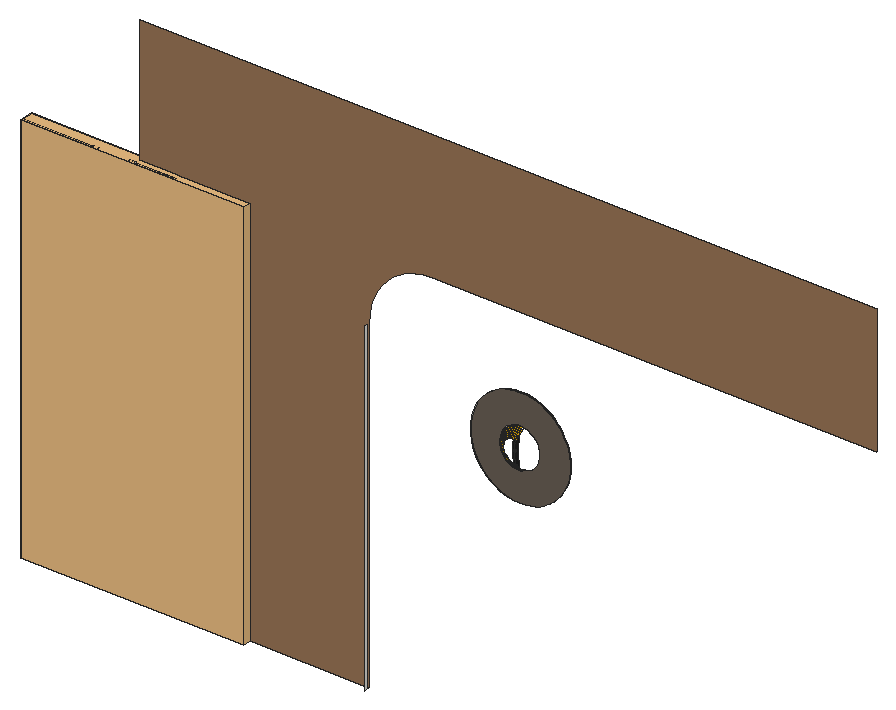
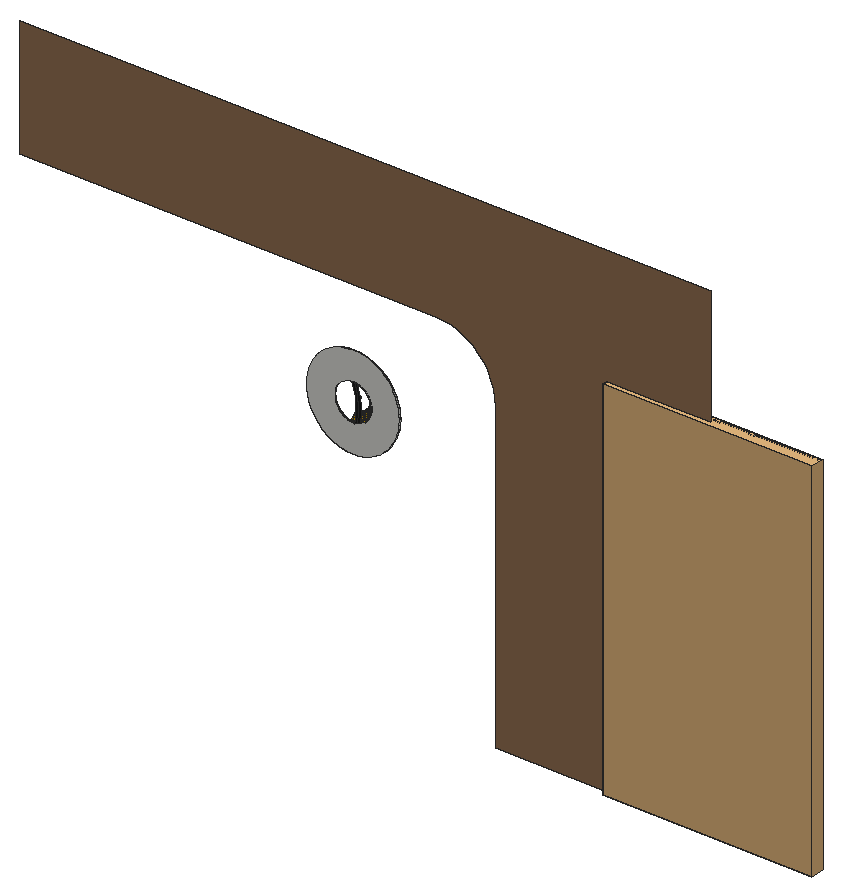
# SketchUp Ruby script. Lengths in inches.
U = 1.inch
M = Sketchup.active_model
def pt(a) = Geom::Point3d.new(a.map { |v| v * U })
def face(e, loops, mat)
  f = e.add_face(loops[0].map { |a| pt(a) })
  loops[1..].each { |l| e.add_face(l.map { |a| pt(a) }).erase! }
  f.material = f.back_material = mat if mat
  f
end
# faces: each face lists its corners as indices into pts; further lists are holes
def faces(e, pts, list, mat = nil) = list.each { |f| face(e, (f[0].is_a?(Array) ? f : [f]).map { |l| l.map { |i| pts[i] } }, mat) }
# xy, xz, yz: faces in a plane at the given z, y or x. An outline is a flat list of corners, or four numbers for a rectangle; further outlines are holes
def ring(l) = l.size == 4 ? [[l[0], l[1]], [l[2], l[1]], [l[2], l[3]], [l[0], l[3]]] : l.each_slice(2).to_a
def flat(e, list, mat, &to3) = list.each { |f| face(e, (f[0].is_a?(Array) ? f : [f]).map { |l| ring(l).map { |u, v| to3.(u, v) } }, mat) }
def xy(e, z, list, mat = nil) = flat(e, list, mat) { |x, y| [x, y, z] }
def xz(e, y, list, mat = nil) = flat(e, list, mat) { |x, z| [x, y, z] }
def yz(e, x, list, mat = nil) = flat(e, list, mat) { |y, z| [x, y, z] }
def lines(e, pts, list) = list.each { |a, b| e.add_line(pt(pts[a]), pt(pts[b])) }
# prism: a flat outline (further loops are holes) pulled along v
def prism(e, loops, v, mat = nil)
  f = face(e, loops, mat); d = Geom::Vector3d.new(v.map { |x| x * U })
  f.pushpull(f.normal.samedirection?(d) ? d.length : -d.length)
end
def box(e, o, s, mat = nil) = prism(e, [[o, [o[0] + s[0], o[1], o[2]], [o[0] + s[0], o[1] + s[1], o[2]], [o[0], o[1] + s[1], o[2]]]], [0, 0, s[2]], mat)
def at(x, y, z, deg = 0) = Geom::Transformation.translation(pt([x, y, z])) * Geom::Transformation.rotation(ORIGIN, Z_AXIS, deg.degrees)
def axes(o, x, y, z) = Geom::Transformation.new([*x, 0, *y, 0, *z, 0, *pt(o).to_a, 1])
def part(name) = M.definitions.add(name)
# library, detail: a bought-in or finely detailed component or shape, given as its bounding box
def library(name, o, s) = part(name).tap { |d| box(d.entities, o, s) }
def detail(e, o, s) = box(e.add_group.entities, o, s)
def put(e, d, t, mat = nil) = e.add_instance(d, t).tap { |i| i.material = mat if mat }
def group(e, t, mat = nil) = e.add_group.tap { |g| g.transformation = t; g.material = mat if mat }.entities
root = M.entities
M.materials.add("Screen Shot 2016-03-02 at 11.42.45 AM").color = [104, 95, 84]
M.materials.add("[0129_WhiteSmoke]").color = [245, 245, 245]
M.materials.add("[0130_Gainsboro]").color = [220, 220, 220]
M.materials.add("[Color D06]").color = [204, 153, 0]
M.materials.add("[Color M08]").color = [30, 30, 30]
M.materials.add("[Wood Floor]").color = [153, 117, 86]
c1 = library("Group\#223",[-0.5,-0.5,0],[45.61,2.875,80.22])
xz(root,755.25,[[[107.55,91.99,108.61,92.04,109.66,92.21,110.6875,92.48,111.68,92.86,112.63,93.35,113.52,93.92,114.34,94.59,115.1,95.34,115.76,96.17,116.34,97.0625,116.83,98.01,117.21,99,117.48,100.03,117.65,101.08,117.7,102.14,117.65,103.2,117.48,104.25,117.21,105.28,116.83,106.27,116.34,107.21,115.76,108.11,115.1,108.93,114.34,109.68,113.52,110.35,112.63,110.93,111.68,111.41,110.6875,111.79,109.66,112.07,108.61,112.24,107.55,112.29,106.49,112.24,105.44,112.07,104.41,111.79,103.42,111.41,102.47,110.93,101.58,110.35,100.76,109.68,100.01,108.93,99.34,108.11,98.76,107.21,98.28,106.27,97.89,105.28,97.62,104.25,97.45,103.2,97.4,102.14,97.45,101.08,97.62,100.03,97.89,99,98.28,98.01,98.76,97.0625,99.34,96.17,100.01,95.34,100.76,94.59,101.58,93.92,102.47,93.35,103.42,92.86,104.41,92.48,105.44,92.21,106.49,92.04],[107.55,98.08,107.125,98.1,106.71,98.17,106.3,98.28,105.9,98.43,105.52,98.62,105.16,98.85,104.83,99.12,104.53,99.42,104.26,99.75,104.03,100.11,103.84,100.49,103.6875,100.88,103.58,101.29,103.51,101.71,103.49,102.14,103.51,102.5625,103.58,102.98,103.6875,103.39,103.84,103.79,104.03,104.17,104.26,104.53,104.53,104.86,104.83,105.16,105.16,105.42,105.52,105.66,105.9,105.85,106.3,106,106.71,106.11,107.125,106.18,107.55,106.2,107.98,106.18,108.39,106.11,108.81,106,109.2,105.85,109.58,105.66,109.9375,105.42,110.27,105.16,110.57,104.86,110.84,104.53,111.07,104.17,111.26,103.79,111.41,103.39,111.52,102.98,111.59,102.5625,111.61,102.14,111.59,101.71,111.52,101.29,111.41,100.88,111.26,100.49,111.07,100.11,110.84,99.75,110.57,99.42,110.27,99.12,109.9375,98.85,109.58,98.62,109.2,98.43,108.81,98.28,108.39,98.17,107.98,98.1]]],"Screen Shot 2016-03-02 at 11.42.45 AM")
xz(root,755.5,[[[107.55,91.99,108.61,92.04,108.73,92.06,109.14,92.125,109.66,92.21,109.77,92.24,110.6875,92.48,111.68,92.86,112.63,93.35,113.4,93.85,113.52,93.92,114.05,94.36,114.34,94.59,115.1,95.34,115.76,96.17,116.34,97.0625,116.83,98.01,117.21,99,117.48,100.03,117.65,101.08,117.7,102.14,117.65,103.2,117.48,104.25,117.21,105.28,116.83,106.27,116.34,107.21,115.76,108.11,115.19,108.8125,115.1,108.93,114.62,109.41,114.34,109.68,113.52,110.35,112.63,110.93,111.68,111.41,111.28,111.57,110.69,111.79,110.6875,111.79,110.29,111.9,109.66,112.07,108.61,112.24,107.55,112.29,106.49,112.24,105.44,112.07,104.41,111.79,103.42,111.41,102.47,110.93,101.58,110.35,100.76,109.68,100.01,108.93,99.34,108.11,98.76,107.21,98.28,106.27,97.89,105.28,97.62,104.25,97.45,103.2,97.4,102.14,97.45,101.08,97.62,100.03,97.89,99,98.28,98.01,98.76,97.0625,99.34,96.17,100.01,95.34,100.76,94.59,101.58,93.92,102.47,93.35,103.42,92.86,104.41,92.48,105.44,92.21,106.49,92.04],[107.55,98.08,107.14,98.1,107.125,98.1,106.71,98.17,106.53,98.21,106.3,98.28,106.125,98.34,105.9,98.43,105.52,98.62,105.16,98.85,104.83,99.12,104.53,99.42,104.26,99.75,104.03,100.11,103.84,100.49,103.6875,100.88,103.58,101.29,103.51,101.71,103.49,102.14,103.51,102.5625,103.58,102.98,103.6875,103.39,103.84,103.79,104.03,104.17,104.26,104.53,104.53,104.86,104.83,105.16,105.16,105.42,105.52,105.66,105.9,105.85,106.3,106,106.71,106.11,106.75,106.12,107.125,106.18,107.16,106.18,107.55,106.2,107.76,106.1875,107.98,106.18,108.39,106.11,108.81,106,109.2,105.85,109.58,105.66,109.9375,105.42,110.27,105.16,110.57,104.86,110.84,104.53,111.07,104.17,111.26,103.79,111.41,103.39,111.52,102.98,111.57,102.66,111.62,102.65,111.59,102.46,111.61,102.14,111.59,101.71,111.52,101.29,111.5,101.21,111.41,100.88,111.26,100.49,111.07,100.11,110.84,99.75,110.76,99.65,110.57,99.42,110.27,99.12,109.9375,98.85,109.58,98.62,109.2,98.43,108.81,98.28,108.39,98.17,107.98,98.1]]])
xz(root,755.5,[[6,46.28,19.81,126.5],[20.99,46.28,27.26,126.5]],"[0129_WhiteSmoke]")
xz(root,755.5,[[28.49,46.28,50.61,46.28,50.61,111.88,50.49,113.79,50.11,115.67,49.5,117.48,48.65,119.19,47.59,120.78,46.33,122.22,44.89,123.48,43.3,124.54,41.59,125.39,39.77,126.01,37.9,126.38,35.99,126.5,28.49,126.5]],"[0130_Gainsboro]")
xz(root,755.5,[[108.73,92.06,109.14,92.125,108.67,92.78,107.875,94.17,107.23,95.63,106.75,97.15,106.53,98.21,106.3,98.28,106.125,98.34,106.39,97.06,106.89,95.5,107.55,94,108.36,92.58],[109.14,92.125,109.66,92.21,109.77,92.24,109.15,93.09,108.39,94.43,107.77,95.84,107.3,97.3,107.14,98.1,107.125,98.1,106.71,98.17,106.53,98.21,106.75,97.15,107.23,95.63,107.875,94.17,108.67,92.78],[107.125,98.1,107.14,98.1,106.99,98.81,106.84,100.34,106.84,101.87,107.01,103.4,107.34,104.9,107.76,106.1875,107.55,106.2,107.16,106.18,106.78,105.05,106.44,103.49,106.27,101.91,106.26,100.31,106.42,98.72,106.53,98.21,106.71,98.17],[106.53,98.21,106.42,98.72,106.26,100.31,106.27,101.91,106.44,103.49,106.78,105.05,107.16,106.18,107.125,106.18,106.75,106.12,106.43,105.15,106.08,103.55,105.9,101.93,105.89,100.29,106.06,98.66,106.125,98.34,106.3,98.28]],"[Color M08]")
xz(root,755.8125,[[19.81,46.28,20.99,126.5],[27.26,46.28,28.49,126.5]],"[Color D06]")
xz(root,756.6875,[[50.61,46.28,75.46,46.28,75.46,113.03,75.57,114.73,75.9,116.39,76.45,118,77.2,119.53,78.14,120.94,79.26,122.22,80.54,123.34,81.96,124.29,83.48,125.04,85.09,125.59,86.76,125.92,88.46,126.03,179.22,126.03,179.22,152.12,28.49,152.12,28.49,126.5,35.99,126.5,37.9,126.38,39.77,126.01,41.59,125.39,43.3,124.54,44.89,123.48,46.33,122.22,47.59,120.78,48.65,119.19,49.5,117.48,50.11,115.67,50.49,113.79,50.61,111.88]],"[Wood Floor]")
yz(root,19.81,[[755.5,46.28,755.8125,126.5]])
yz(root,20.99,[[755.5,46.28,755.8125,126.5]])
yz(root,27.26,[[755.5,46.28,755.8125,126.5]])
yz(root,28.49,[[755.5,46.28,755.8125,126.5]])
yz(root,75.46,[[755.5,46.28,756.09,113.03]])
p = [[105.44,755.5,92.21],[106.49,755.5,92.04],[106.49,755.25,92.04],[105.44,755.25,92.21],[107.55,755.5,91.99],[107.55,755.25,91.99],
  [108.61,755.5,92.04],[108.61,755.25,92.04],[104.41,755.5,92.48],[104.41,755.25,92.48],[103.42,755.5,92.86],[103.42,755.25,92.86],
  [102.47,755.5,93.35],[102.47,755.25,93.35],[101.58,755.5,93.92],[101.58,755.25,93.92],[100.76,755.5,94.59],[100.76,755.25,94.59],
  [100.01,755.5,95.34],[100.01,755.25,95.34],[99.34,755.5,96.17],[99.34,755.25,96.17],[98.76,755.5,97.0625],[98.76,755.25,97.0625],
  [98.28,755.5,98.01],[98.28,755.25,98.01],[97.89,755.5,99],[97.89,755.25,99],[107.125,755.25,98.1],[107.15,754.91,98.3],
  [106.75,754.91,98.37],[106.71,755.25,98.17],[107.55,755.25,98.08],[107.55,754.91,98.28],[107.98,755.25,98.1],[107.95,754.91,98.3],
  [107.125,755.5,98.1],[106.71,755.5,98.17],[107.55,755.5,98.08],[107.14,755.5,98.1],[107.98,755.5,98.1],[106.36,754.91,98.47],
  [106.3,755.25,98.28],[106.53,755.5,98.21],[106.3,755.5,98.28],[107.17,754.6,98.55],[106.8,754.6,98.61],[107.55,754.6,98.53],
  [107.93,754.6,98.55],[108.35,754.91,98.37],[108.3,754.6,98.61],[105.98,754.91,98.62],[105.9,755.25,98.43],[106.125,755.5,98.34],
  [105.9,755.5,98.43],[106.44,754.6,98.71],[105.62,754.91,98.8],[105.52,755.25,98.62],[105.52,755.5,98.62],[107.2,754.33,98.83],
  [106.86,754.33,98.88],[107.55,754.33,98.8125],[107.9,754.33,98.83],[108.24,754.33,98.88],[106.08,754.6,98.84],[106.52,754.33,98.97],
  [105.75,754.6,99.01],[105.28,754.91,99.02],[105.16,755.25,98.85],[105.16,755.5,98.85],[106.2,754.33,99.1],[107.24,754.09,99.14],
  [106.92,754.09,99.19],[107.55,754.09,99.125],[107.87,754.09,99.14],[108.18,754.09,99.19],[105.89,754.33,99.26],[105.43,754.6,99.22],
  [106.62,754.09,99.27],[104.97,754.91,99.27],[104.83,755.25,99.12],[104.83,755.5,99.12],[106.33,754.09,99.39],[105.6,754.33,99.45],
  [105.14,754.6,99.46],[97.62,755.5,100.03],[97.62,755.25,100.03],[107.27,753.9,99.48],[107,753.9,99.53],[107.55,753.9,99.47],
  [107.83,753.9,99.48],[108.11,753.9,99.53],[106.04,754.09,99.53],[104.69,754.91,99.56],[104.53,755.25,99.42],[104.53,755.5,99.42],
  [106.73,753.9,99.6],[105.32,754.33,99.67],[106.46,753.9,99.7],[105.78,754.09,99.7],[104.87,754.6,99.72],[106.22,753.9,99.83],
  [105.54,754.09,99.9],[104.43,754.91,99.87],[104.26,755.25,99.75],[104.26,755.5,99.75],[107.07,753.75,99.88],[106.84,753.75,99.94],
  [107.31,753.75,99.84],[107.55,753.75,99.83],[107.79,753.75,99.84],[108.03,753.75,99.88],[105.98,753.9,99.98],[105.08,754.33,99.91],
  [106.61,753.75,100.03],[104.63,754.6,100.02],[106.4,753.75,100.14],[105.76,753.9,100.15],[105.3125,754.09,100.12],[104.86,754.33,100.18],
  [106.19,753.75,100.27],[104.21,754.91,100.21],[104.03,755.25,100.11],[104.03,755.5,100.11],[105.57,753.9,100.35],[105.11,754.09,100.37],
  [104.42,754.6,100.33],[106.01,753.75,100.42],[104.67,754.33,100.47],[97.45,755.5,101.08],[97.45,755.25,101.08],[105.39,753.9,100.57],
  [104.03,754.91,100.57],[103.84,755.25,100.49],[103.84,755.5,100.49],[105.84,753.75,100.59],[104.94,754.09,100.63],[104.25,754.6,100.67],
  [104.51,754.33,100.78],[105.68,753.75,100.78],[105.24,753.9,100.8],[104.8,754.09,100.91],[103.88,754.91,100.95],[103.6875,755.25,100.88],
  [103.6875,755.5,100.88],[105.55,753.75,100.98],[105.11,753.9,101.05],[104.12,754.6,101.02],[104.39,754.33,101.11],[105.44,753.75,101.2],
  [104.6875,754.09,101.21],[105.01,753.9,101.3125],[104.02,754.6,101.39],[103.78,754.91,101.34],[103.58,755.25,101.29],[103.58,755.5,101.29],
  [104.3,754.33,101.45],[105.36,753.75,101.43],[104.6,754.09,101.51],[97.4,755.5,102.14],[97.4,755.25,102.14],[104.9375,753.9,101.58],
  [105.29,753.75,101.66],[103.96,754.6,101.76],[103.72,754.91,101.74],[103.51,755.25,101.71],[103.51,755.5,101.71],[104.55,754.09,101.82],
  [104.24,754.33,101.79],[104.89,753.9,101.86],[105.26,753.75,101.9],[103.94,754.6,102.14],[103.69,754.91,102.14],[103.49,755.25,102.14],
  [103.49,755.5,102.14],[104.88,753.9,102.14],[104.54,754.09,102.14],[104.22,754.33,102.14],[105.24,753.75,102.14],[105.26,753.75,102.38],
  [104.89,753.9,102.42],[107.18,753.71,102.14],[107.55,753.85,102.14],[107.18,753.71,102.18],[107.19,753.71,102.21],[107.2,753.71,102.25],
  [107.21,753.71,102.29],[107.23,753.71,102.32],[107.25,753.71,102.35],[107.28,753.71,102.38],[107.3,753.71,102.41],[107.33,753.71,102.4375],
  [107.37,753.71,102.46],[107.4,753.71,102.47],[107.4375,753.71,102.49],[107.47,753.71,102.5],[107.51,753.71,102.5],[107.55,753.71,102.51],
  [107.73,753.71,102.46],[107.77,753.71,102.4375],[107.8,753.71,102.41],[107.82,753.71,102.38],[107.85,753.71,102.35],[107.87,753.71,102.32],
  [107.89,753.71,102.29],[107.9,753.71,102.25],[107.91,753.71,102.21],[107.92,753.71,102.18],[107.92,753.71,102.14],[104.55,754.09,102.45],
  [104.24,754.33,102.49],[103.96,754.6,102.52],[103.72,754.91,102.54],[103.51,755.25,102.5625],[97.45,755.5,103.2],[97.45,755.25,103.2],
  [103.51,755.5,102.5625],[105.29,753.75,102.62],[104.9375,753.9,102.69],[104.6,754.09,102.76],[104.3,754.33,102.83],[104.02,754.6,102.89],
  [103.78,754.91,102.94],[103.58,755.25,102.98],[105.36,753.75,102.85],[105.01,753.9,102.96],[103.58,755.5,102.98],[104.6875,754.09,103.07],
  [104.39,754.33,103.17],[104.12,754.6,103.25],[105.44,753.75,103.08],[105.11,753.9,103.22],[103.88,754.91,103.33],[103.6875,755.25,103.39],
  [104.8,754.09,103.36],[103.6875,755.5,103.39],[105.55,753.75,103.29],[105.24,753.9,103.47],[104.51,754.33,103.49],[104.94,754.09,103.64],
  [104.25,754.6,103.61],[97.62,755.5,104.25],[97.62,755.25,104.25],[105.68,753.75,103.49],[105.39,753.9,103.71],[104.03,754.91,103.71],
  [103.84,755.25,103.79],[104.67,754.33,103.8],[103.84,755.5,103.79],[105.84,753.75,103.68],[105.57,753.9,103.92],[105.11,754.09,103.91],
  [104.42,754.6,103.94],[104.86,754.33,104.09],[104.21,754.91,104.07],[106.01,753.75,103.85],[105.76,753.9,104.12],[105.3125,754.09,104.15],
  [104.03,755.25,104.17],[104.63,754.6,104.26],[104.03,755.5,104.17],[106.19,753.75,104],[105.98,753.9,104.3],[105.54,754.09,104.375],
  [105.08,754.33,104.36],[104.43,754.91,104.4],[106.4,753.75,104.14],[106.22,753.9,104.45],[106.61,753.75,104.25],[106.46,753.9,104.58],
  [105.78,754.09,104.57],[104.87,754.6,104.55],[104.26,755.25,104.53],[106.84,753.75,104.33],[106.73,753.9,104.68],[105.32,754.33,104.61],
  [97.89,755.5,105.28],[97.89,755.25,105.28],[104.26,755.5,104.53],[107.07,753.75,104.39],[107,753.9,104.75],[106.04,754.09,104.75],
  [104.69,754.91,104.72],[107.31,753.75,104.43],[107.27,753.9,104.79],[107.55,753.75,104.44],[107.55,753.9,104.81],[107.79,753.75,104.43],
  [107.83,753.9,104.79],[108.03,753.75,104.39],[108.11,753.9,104.75],[105.6,754.33,104.83],[105.14,754.6,104.82],[104.53,755.25,104.86],
  [106.33,754.09,104.89],[104.53,755.5,104.86],[106.62,754.09,105],[105.89,754.33,105.02],[105.43,754.6,105.06],[104.97,754.91,105],
  [106.92,754.09,105.08],[107.24,754.09,105.13],[107.87,754.09,105.13],[108.18,754.09,105.08],[106.2,754.33,105.18],[104.83,755.25,105.16],
  [107.55,754.09,105.15],[105.75,754.6,105.26],[105.28,754.91,105.26],[106.52,754.33,105.3],[104.83,755.5,105.16],[106.86,754.33,105.39],
  [106.08,754.6,105.44],[105.16,755.25,105.42],[107.2,754.33,105.45],[107.55,754.33,105.46],[107.9,754.33,105.45],[108.24,754.33,105.39],
  [105.62,754.91,105.48],[106.44,754.6,105.57],[105.16,755.5,105.42],[106.8,754.6,105.67],[105.98,754.91,105.66],[105.52,755.25,105.66],
  [98.28,755.5,106.27],[98.28,755.25,106.27],[107.17,754.6,105.73],[107.55,754.6,105.75],[107.93,754.6,105.73],[108.3,754.6,105.67],
  [106.36,754.91,105.8],[105.52,755.5,105.66],[105.9,755.25,105.85],[106.75,754.91,105.91],[107.15,754.91,105.97],[107.55,754.91,105.99],
  [107.95,754.91,105.97],[108.35,754.91,105.91],[106.3,755.25,106],[105.9,755.5,105.85],[106.71,755.25,106.11],[106.3,755.5,106],
  [107.125,755.25,106.18],[107.55,755.25,106.2],[107.98,755.25,106.18],[106.71,755.5,106.11],[106.75,755.5,106.12],[107.125,755.5,106.18],
  [107.16,755.5,106.18],[107.55,755.5,106.2],[107.76,755.5,106.1875],[107.98,755.5,106.18],[98.76,755.5,107.21],[98.76,755.25,107.21]]
faces(root,p,[[0,1,2,3],[1,4,5,2],[4,6,7,5],[8,0,3,9],[10,8,9,11],[12,10,11,13],[14,12,13,15],[16,14,15,17],
  [18,16,17,19],[20,18,19,21],[22,20,21,23],[24,22,23,25],[26,24,25,27],[36,37,31,28],[38,39,36,28,32],[40,38,32,34],
  [37,43,44,42,31],[44,53,54,52,42],[54,58,57,52],[58,69,68,57],[69,81,80,68],[85,26,27,86],[81,95,94,80],[95,105,104,94],
  [105,123,122,104],[129,85,86,130],[123,134,133,122],[134,144,143,133],[144,155,154,143],[159,129,130,160],[155,166,165,154],[166,174,173,165],
  [214,159,160,215],[174,216,213,173],[216,226,223,213],[226,235,233,223],[241,214,215,242],[235,248,246,233],[248,260,258,246],[276,241,242,277],
  [260,278,272,258],[278,295,293,272],[295,310,305,293],[310,320,313,305],[324,276,277,325],[320,331,323,313],[331,339,332,323],[339,341,338,332],
  [341,345,340,338],[345,346,347,342,340],[347,348,349,343,342],[349,350,351,344,343],[352,324,325,353]])
faces(root,p,[[28,29,30,31],[32,33,29,28],[34,35,33,32],[31,30,41,42],[29,45,46,30],[33,47,45,29],[35,48,47,33],[49,50,48,35],
  [42,41,51,52],[30,46,55,41],[52,51,56,57],[45,59,60,46],[47,61,59,45],[48,62,61,47],[50,63,62,48],[41,55,64,51],
  [46,60,65,55],[51,64,66,56],[57,56,67,68],[55,65,70,64],[59,71,72,60],[61,73,71,59],[62,74,73,61],[63,75,74,62],
  [64,70,76,66],[56,66,77,67],[60,72,78,65],[68,67,79,80],[65,78,82,70],[66,76,83,77],[67,77,84,79],[71,87,88,72],
  [73,89,87,71],[74,90,89,73],[75,91,90,74],[70,82,92,76],[80,79,93,94],[72,88,96,78],[77,83,97,84],[78,96,98,82],
  [76,92,99,83],[79,84,100,93],[82,98,101,92],[83,99,102,97],[94,93,103,104],[88,106,107,96],[87,108,106,88],[89,109,108,87],
  [90,110,109,89],[91,111,110,90],[92,101,112,99],[84,97,113,100],[96,107,114,98],[93,100,115,103],[98,114,116,101],[99,112,117,102],
  [97,102,118,113],[100,113,119,115],[101,116,120,112],[104,103,121,122],[102,117,124,118],[113,118,125,119],[103,115,126,121],[112,120,127,117],
  [115,119,128,126],[118,124,131,125],[122,121,132,133],[117,127,135,124],[119,125,136,128],[121,126,137,132],[126,128,138,137],[124,135,139,131],
  [125,131,140,136],[128,136,141,138],[133,132,142,143],[131,139,145,140],[136,140,146,141],[132,137,147,142],[137,138,148,147],[140,145,149,146],
  [138,141,150,148],[141,146,151,150],[142,147,152,153],[143,142,153,154],[147,148,156,152],[146,149,157,151],[148,150,158,156],[150,151,161,158],
  [151,157,162,161],[153,152,163,164],[154,153,164,165],[156,158,167,168],[152,156,168,163],[158,161,169,167],[161,162,170,169],[164,163,171,172],
  [165,164,172,173],[167,169,175,176],[168,167,176,177],[163,168,177,171],[169,170,178,175],[175,178,179,180],[181,182,183],[183,182,184],
  [184,182,185],[185,182,186],[186,182,187],[187,182,188],[188,182,189],[189,182,190],[190,182,191],[191,182,192],
  [192,182,193],[193,182,194],[194,182,195],[195,182,196],[196,182,197],[198,182,199],[199,182,200],[201,182,202],
  [202,182,203],[203,182,204],[204,182,205],[205,182,206],[206,182,207],[207,182,208],[176,175,180,209],[177,176,209,210],
  [171,177,210,211],[172,171,211,212],[173,172,212,213],[180,179,217,218],[209,180,218,219],[210,209,219,220],[211,210,220,221],[212,211,221,222],
  [213,212,222,223],[218,217,224,225],[219,218,225,227],[220,219,227,228],[221,220,228,229],[225,224,230,231],[222,221,229,232],[223,222,232,233],
  [227,225,231,234],[231,230,236,237],[228,227,234,238],[234,231,237,239],[229,228,238,240],[237,236,243,244],[232,229,240,245],[233,232,245,246],
  [238,234,239,247],[244,243,249,250],[239,237,244,251],[240,238,247,252],[247,239,251,253],[245,240,252,254],[250,249,255,256],[251,244,250,257],
  [246,245,254,258],[252,247,253,259],[256,255,261,262],[257,250,256,263],[253,251,257,264],[254,252,259,265],[262,261,266,267],[267,266,268,269],
  [263,256,262,270],[259,253,264,271],[258,254,265,272],[269,268,273,274],[264,257,263,275],[274,273,279,280],[270,262,267,281],[265,259,271,282],
  [280,279,283,284],[284,283,285,286],[286,285,287,288],[288,287,289,290],[275,263,270,291],[271,264,275,292],[272,265,282,293],[281,267,269,294],
  [294,269,274,296],[291,270,281,297],[292,275,291,298],[282,271,292,299],[296,274,280,300],[300,280,284,301],[302,288,290,303],[297,281,294,304],
  [293,282,299,305],[301,284,286,306],[306,286,288,302],[298,291,297,307],[299,292,298,308],[304,294,296,309],[309,296,300,311],[307,297,304,312],
  [305,299,308,313],[311,300,301,314],[314,301,306,315],[315,306,302,316],[316,302,303,317],[308,298,307,318],[312,304,309,319],[319,309,311,321],
  [318,307,312,322],[313,308,318,323],[321,311,314,326],[326,314,315,327],[327,315,316,328],[328,316,317,329],[322,312,319,330],[323,318,322,332],
  [330,319,321,333],[333,321,326,334],[334,326,327,335],[335,327,328,336],[336,328,329,337],[332,322,330,338],[338,330,333,340],[340,333,334,342],
  [342,334,335,343],[343,335,336,344]],"[Color D06]")
put(root,c1,at(6,755.5,46.28))
